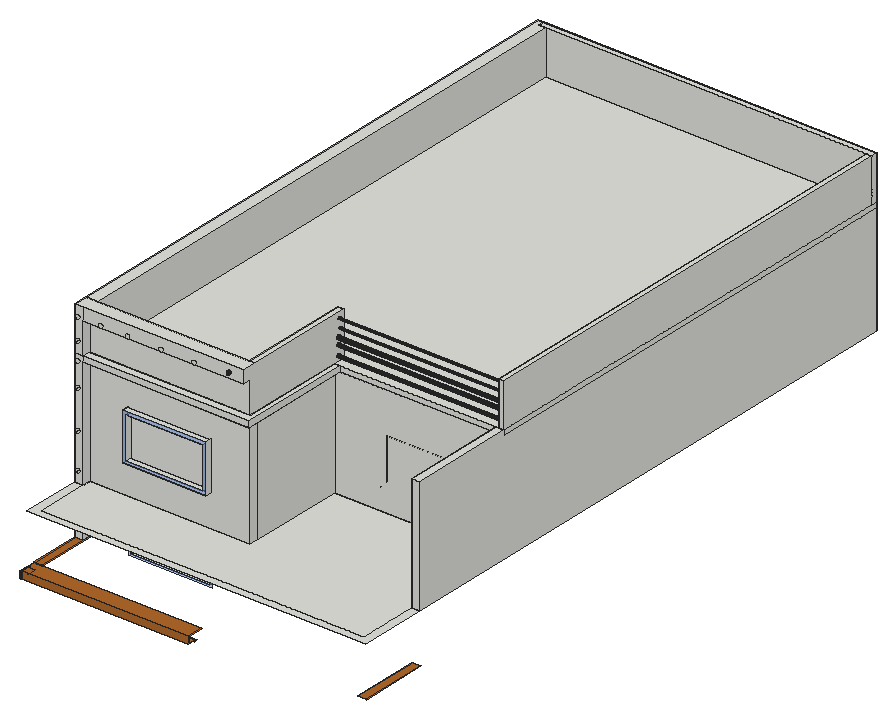
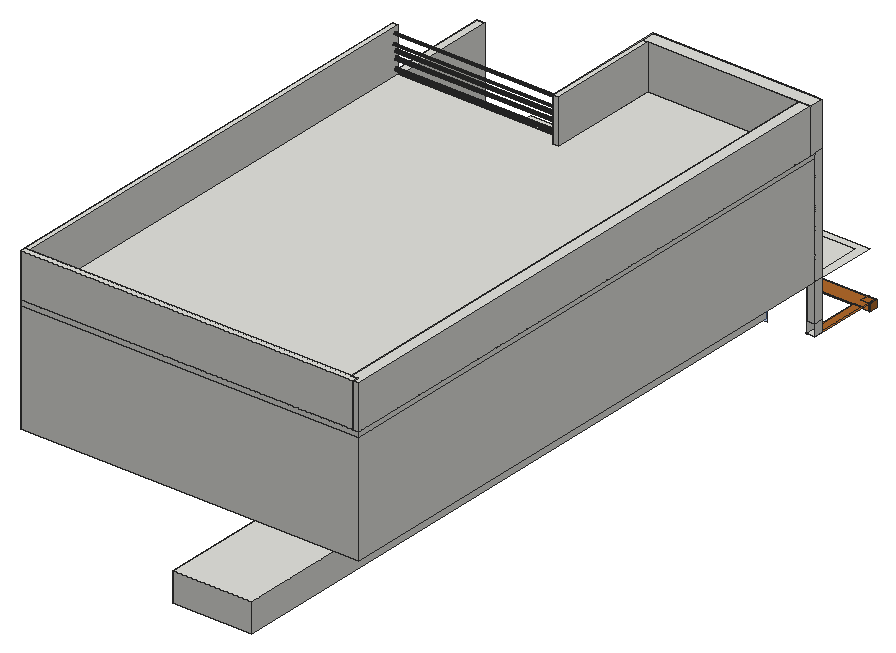
# SketchUp Ruby script. Lengths in inches.
U = 1.inch
M = Sketchup.active_model
def pt(a) = Geom::Point3d.new(a.map { |v| v * U })
def face(e, loops, mat)
  f = e.add_face(loops[0].map { |a| pt(a) })
  loops[1..].each { |l| e.add_face(l.map { |a| pt(a) }).erase! }
  f.material = f.back_material = mat if mat
  f
end
# faces: each face lists its corners as indices into pts; further lists are holes
def faces(e, pts, list, mat = nil) = list.each { |f| face(e, (f[0].is_a?(Array) ? f : [f]).map { |l| l.map { |i| pts[i] } }, mat) }
# xy, xz, yz: faces in a plane at the given z, y or x. An outline is a flat list of corners, or four numbers for a rectangle; further outlines are holes
def ring(l) = l.size == 4 ? [[l[0], l[1]], [l[2], l[1]], [l[2], l[3]], [l[0], l[3]]] : l.each_slice(2).to_a
def flat(e, list, mat, &to3) = list.each { |f| face(e, (f[0].is_a?(Array) ? f : [f]).map { |l| ring(l).map { |u, v| to3.(u, v) } }, mat) }
def xy(e, z, list, mat = nil) = flat(e, list, mat) { |x, y| [x, y, z] }
def xz(e, y, list, mat = nil) = flat(e, list, mat) { |x, z| [x, y, z] }
def yz(e, x, list, mat = nil) = flat(e, list, mat) { |y, z| [x, y, z] }
def lines(e, pts, list) = list.each { |a, b| e.add_line(pt(pts[a]), pt(pts[b])) }
# prism: a flat outline (further loops are holes) pulled along v
def prism(e, loops, v, mat = nil)
  f = face(e, loops, mat); d = Geom::Vector3d.new(v.map { |x| x * U })
  f.pushpull(f.normal.samedirection?(d) ? d.length : -d.length)
end
def box(e, o, s, mat = nil) = prism(e, [[o, [o[0] + s[0], o[1], o[2]], [o[0] + s[0], o[1] + s[1], o[2]], [o[0], o[1] + s[1], o[2]]]], [0, 0, s[2]], mat)
def at(x, y, z, deg = 0) = Geom::Transformation.translation(pt([x, y, z])) * Geom::Transformation.rotation(ORIGIN, Z_AXIS, deg.degrees)
def axes(o, x, y, z) = Geom::Transformation.new([*x, 0, *y, 0, *z, 0, *pt(o).to_a, 1])
def part(name) = M.definitions.add(name)
# library, detail: a bought-in or finely detailed component or shape, given as its bounding box
def library(name, o, s) = part(name).tap { |d| box(d.entities, o, s) }
def detail(e, o, s) = box(e.add_group.entities, o, s)
def put(e, d, t, mat = nil) = e.add_instance(d, t).tap { |i| i.material = mat if mat }
def group(e, t, mat = nil) = e.add_group.tap { |g| g.transformation = t; g.material = mat if mat }.entities
root = M.entities
M.materials.add("[Translucent Glass Blue]").color = [100, 149, 237]
M.materials["[Translucent Glass Blue]"].alpha = 0.5
M.materials.add("[Wood Bamboo]").color = [177, 105, 43]
c1 = part("Component\#1")
xy(c1.entities,0,[[0,0,369,0,369,74,360,74,360,9,9,9,9,74,0,74],[9,9,360,9,360,189,184,189,184,74,9,74],[0,74,184,74,184,83,9,83,9,687,360,687,360,198,175.5625,198,175.5625,189,360,189,360,74,369,74,369,696,0,696],[9,83,175,83,175,198,360,198,360,687,9,687],[175,189,175.5625,198]])
xy(c1.entities,120,[[0,74,184,83],[0,83,9,189],[9,83,9,687,360,687,360,198,175.5625,198,175.5625,189,175,189,175,83],[0,189,9,696],[175.5625,189,369,198],
  [360,198,369,696],[9,687,360,696]])
xy(c1.entities,126,[[0,74,184,74,184,189,369,189,369,696,0,696],[360,74,369,189]])
xz(c1.entities,74,[[0,0,9,120],[9,0,184,120],[360,0,369,126],[0,120,184,126]])
xz(c1.entities,83,[[9,0,175,120],[175,0,184,120]])
xz(c1.entities,189,[[175,0,175.5625,120],[175.5625,0,184,120],[184,0,360,120],[184,120,360,126],[360,120,369,126]])
xz(c1.entities,198,[[175.5625,0,360,120]])
xz(c1.entities,687,[[9,0,360,120]])
xz(c1.entities,696,[[0,0,369,120],[0,120,369,126]])
yz(c1.entities,0,[[74,0,696,120],[74,120,696,126]])
yz(c1.entities,9,[[83,0,687,120]])
yz(c1.entities,175,[[83,0,189,120]])
yz(c1.entities,175.5625,[[189,0,198,120]])
yz(c1.entities,184,[[74,0,83,120],[83,0,189,120],[74,120,189,126]])
yz(c1.entities,360,[[74,0,189,126],[198,0,687,120]])
yz(c1.entities,369,[[74,0,696,0,696,120,189,120,189,126,74,126],[189,120,696,126]])
xy(root,62.76,[[157.01,36.81,183.01,40.24]],"[Wood Bamboo]")
xy(root,64.47,[[0.51,27.81,1.51,36.81],[1.51,27.81,1.51,36.81,83.28,36.81,83.28,45.81,141.28,45.81,141.28,36.81,183.01,36.81,183.01,27.81],[183.01,27.81,184.01,36.81],[82.28,36.81,83.28,45.81],[141.28,36.81,142.28,45.81]],"[Wood Bamboo]")
xy(root,70.55,[[54.61,110.81,140.53,811.24]])
xy(root,72,[[9.45,27.57,9.45,27.59,1.39,27.81,0.51,27.81,0.51,36.81,0.27,27.8125],[10.45,27.57,10.45,27.81,9.45,27.81,9.45,27.59],[9.45,27.59,9.45,27.81,1.39,27.81],[0.51,27.81,1.39,27.81,1.27,27.8125,1.51,36.78,0.51,36.81],[1.39,27.81,1.51,27.81,1.51,36.78,1.27,27.8125],
  [1.51,27.81,9.45,27.81,9.6875,36.5625,1.51,36.78],[10.45,27.81,183.01,27.81,183.01,45.81,1.51,45.81,1.51,36.81,10.6875,36.5625],[9.45,27.81,10.45,27.81,10.6875,36.5625,1.51,36.81,1.51,36.78,9.6875,36.5625],[183.01,27.81,184.01,45.81],[1.51,36.78,1.51,45.81,0.51,45.81,0.51,36.81],
  [360.51,36.81,361.51,110.81],[361.51,36.81,369.51,110.81],[369.51,36.81,370.51,110.81]],"[Wood Bamboo]")
xy(root,72.3125,[[0.51,45.81,1.51,110.81],[1.51,45.81,9.51,110.81],[9.51,45.81,10.51,110.81]],"[Wood Bamboo]")
xy(root,72.54,[[0.51,101.81,9.51,110.81]])
xy(root,84.53,[[0.51,101.81,9.51,110.81]])
xy(root,102.16,[[54.61,110.81,140.53,811.24]])
xy(root,125.75,[[0.51,101.81,9.51,110.81]])
xy(root,126,[[0.51,101.81,9.51,110.81]])
xy(root,156.23,[[241.98,225.81,319.92,292.56]])
xy(root,160.68,[[50.59,104.68,141.46,172.06]])
xy(root,164.35,[[54.26,104.68,137.79,696.81]])
xy(root,201.73,[[241.98,225.81,319.92,292.56]])
xy(root,209.32,[[54.26,104.68,137.79,696.81]])
xy(root,212.99,[[50.59,104.68,141.46,172.06]])
xy(root,246,[[9.51,101.81,190.64,110.81],[184.51,110.81,190.64,225.81]])
xy(root,252,[[0.51,101.81,0.51,116.96,184.51,116.96,184.51,110.81,9.51,110.81,9.51,101.81],[9.51,101.81,190.64,101.81,190.64,225.81,184.51,225.81,184.51,110.81,9.51,110.81],[0.51,116.96,0.51,732.81,6.51,732.81,6.51,726.81,13.58,726.81,13.58,116.96],[178.51,116.96,184.51,237.875],[363.51,225.81,369.51,726.81],
  [6.51,726.81,369.51,732.81]])
xy(root,286.07,[[9.51,101.81,184.51,110.81]])
xy(root,300,[[0.51,101.81,184.51,116.96],[0.51,116.96,13.58,116.96,13.58,726.81,6.51,726.81,6.51,732.81,0.51,732.81],[178.51,116.96,184.51,237.875],[363.51,225.81,369.51,726.81],[6.51,726.81,369.51,732.81]])
xz(root,27.81,[[0.51,64.47,1.51,72],[1.51,64.47,183.01,72],[183.01,64.47,184.01,72]],"[Wood Bamboo]")
xz(root,45.81,[[0.51,72,1.51,72.3125],[1.51,72,9.51,72.3125],[9.51,72,10.51,72.3125]],"[Wood Bamboo]")
xz(root,96.37,[[[7.9375,84.47,8.45,84.53,8.9375,84.73,9.35,85.05,9.67,85.47,9.87,85.95,9.9375,86.47,9.87,86.98,9.67,87.47,9.35,87.88,8.9375,88.2,8.45,88.4,7.9375,88.47,7.42,88.4,6.9375,88.2,6.52,87.88,6.2,87.47,6.01,86.98,5.9375,86.47,6.01,85.95,6.2,85.47,6.52,85.05,6.9375,84.73,7.42,84.53],[7.9375,85.47,7.68,85.5,7.4375,85.6,7.23,85.76,7.07,85.97,6.97,86.21,6.9375,86.47,6.97,86.72,7.07,86.97,7.23,87.17,7.4375,87.33,7.68,87.43,7.9375,87.47,8.2,87.43,8.4375,87.33,8.64,87.17,8.8,86.97,8.9,86.72,8.9375,86.47,8.9,86.21,8.8,85.97,8.64,85.76,8.4375,85.6,8.2,85.5]],[[7.9375,113.05,8.45,113.12,8.9375,113.32,9.35,113.64,9.67,114.05,9.87,114.54,9.9375,115.05,9.87,115.57,9.67,116.05,9.35,116.47,8.9375,116.79,8.45,116.99,7.9375,117.05,7.42,116.99,6.9375,116.79,6.52,116.47,6.2,116.05,6.01,115.57,5.9375,115.05,6.01,114.54,6.2,114.05,6.52,113.64,6.9375,113.32,7.42,113.12],[7.9375,114.05,7.68,114.09,7.4375,114.1875,7.23,114.35,7.07,114.55,6.97,114.8,6.9375,115.05,6.97,115.3125,7.07,115.55,7.23,115.76,7.4375,115.92,7.68,116.02,7.9375,116.05,8.2,116.02,8.4375,115.92,8.64,115.76,8.8,115.55,8.9,115.3125,8.9375,115.05,8.9,114.8,8.8,114.55,8.64,114.35,8.4375,114.1875,8.2,114.09]],[[7.9375,140.18,8.45,140.25,8.9375,140.45,9.35,140.77,9.67,141.18,9.87,141.66,9.9375,142.18,9.87,142.7,9.67,143.18,9.35,143.59,8.9375,143.91,8.45,144.11,7.9375,144.18,7.42,144.11,6.9375,143.91,6.52,143.59,6.2,143.18,6.01,142.7,5.9375,142.18,6.01,141.66,6.2,141.18,6.52,140.77,6.9375,140.45,7.42,140.25],[7.9375,141.18,7.68,141.21,7.4375,141.3125,7.23,141.47,7.07,141.68,6.97,141.92,6.9375,142.18,6.97,142.4375,7.07,142.68,7.23,142.89,7.4375,143.05,7.68,143.15,7.9375,143.18,8.2,143.15,8.4375,143.05,8.64,142.89,8.8,142.68,8.9,142.4375,8.9375,142.18,8.9,141.92,8.8,141.68,8.64,141.47,8.4375,141.3125,8.2,141.21]],[[7.9375,179.1,8.45,179.17,8.9375,179.37,9.35,179.69,9.67,180.1,9.87,180.59,9.9375,181.1,9.87,181.62,9.67,182.1,9.35,182.52,8.9375,182.84,8.45,183.04,7.9375,183.1,7.42,183.04,6.9375,182.84,6.52,182.52,6.2,182.1,6.01,181.62,5.9375,181.1,6.01,180.59,6.2,180.1,6.52,179.69,6.9375,179.37,7.42,179.17],[7.9375,180.1,7.68,180.14,7.4375,180.24,7.23,180.4,7.07,180.6,6.97,180.85,6.9375,181.1,6.97,181.36,7.07,181.6,7.23,181.8125,7.4375,181.97,7.68,182.07,7.9375,182.1,8.2,182.07,8.4375,181.97,8.64,181.8125,8.8,181.6,8.9,181.36,8.9375,181.1,8.9,180.85,8.8,180.6,8.64,180.4,8.4375,180.24,8.2,180.14]],[[7.9375,221.04,8.45,221.11,8.9375,221.31,9.35,221.63,9.67,222.04,9.87,222.52,9.9375,223.04,9.87,223.56,9.67,224.04,9.35,224.46,8.9375,224.77,8.45,224.97,7.9375,225.04,7.42,224.97,6.9375,224.77,6.52,224.46,6.2,224.04,6.01,223.56,5.9375,223.04,6.01,222.52,6.2,222.04,6.52,221.63,6.9375,221.31,7.42,221.11],[7.9375,222.04,7.68,222.08,7.4375,222.18,7.23,222.34,7.07,222.54,6.97,222.78,6.9375,223.04,6.97,223.3,7.07,223.54,7.23,223.75,7.4375,223.91,7.68,224.01,7.9375,224.04,8.2,224.01,8.4375,223.91,8.64,223.75,8.8,223.54,8.9,223.3,8.9375,223.04,8.9,222.78,8.8,222.54,8.64,222.34,8.4375,222.18,8.2,222.08]],
  [[7.9375,247.17,8.45,247.24,8.9375,247.44,9.35,247.75,9.67,248.17,9.87,248.65,9.9375,249.17,9.87,249.68,9.67,250.17,9.35,250.58,8.9375,250.9,8.45,251.1,7.9375,251.17,7.42,251.1,6.9375,250.9,6.52,250.58,6.2,250.17,6.01,249.68,5.9375,249.17,6.01,248.65,6.2,248.17,6.52,247.75,6.9375,247.44,7.42,247.24],[7.9375,248.17,7.68,248.2,7.4375,248.3,7.23,248.46,7.07,248.67,6.97,248.91,6.9375,249.17,6.97,249.43,7.07,249.67,7.23,249.875,7.4375,250.03,7.68,250.13,7.9375,250.17,8.2,250.13,8.4375,250.03,8.64,249.875,8.8,249.67,8.9,249.43,8.9375,249.17,8.9,248.91,8.8,248.67,8.64,248.46,8.4375,248.3,8.2,248.2]],[[7.92,267.07,8.4375,267.14,8.92,267.34,9.33,267.65,9.65,268.07,9.85,268.55,9.92,269.07,9.85,269.59,9.65,270.07,9.33,270.48,8.92,270.8,8.4375,271,7.92,271.07,7.4,271,6.92,270.8,6.51,270.48,6.1875,270.07,5.99,269.59,5.92,269.07,5.99,268.55,6.1875,268.07,6.51,267.65,6.92,267.34,7.4,267.14],[7.92,268.07,7.66,268.1,7.42,268.2,7.21,268.36,7.05,268.57,6.95,268.81,6.92,269.07,6.95,269.33,7.05,269.57,7.21,269.78,7.42,269.93,7.66,270.03,7.92,270.07,8.18,270.03,8.42,269.93,8.63,269.78,8.79,269.57,8.89,269.33,8.92,269.07,8.89,268.81,8.79,268.57,8.63,268.36,8.42,268.2,8.18,268.1]],[[7.92,290.19,8.4375,290.26,8.92,290.46,9.33,290.78,9.65,291.19,9.85,291.68,9.92,292.19,9.85,292.71,9.65,293.19,9.33,293.61,8.92,293.93,8.4375,294.125,7.92,294.19,7.4,294.125,6.92,293.93,6.51,293.61,6.1875,293.19,5.99,292.71,5.92,292.19,5.99,291.68,6.1875,291.19,6.51,290.78,6.92,290.46,7.4,290.26],[7.92,291.19,7.66,291.23,7.42,291.33,7.21,291.49,7.05,291.69,6.95,291.93,6.92,292.19,6.95,292.45,7.05,292.69,7.21,292.9,7.42,293.06,7.66,293.16,7.92,293.19,8.18,293.16,8.42,293.06,8.63,292.9,8.79,292.69,8.89,292.45,8.92,292.19,8.89,291.93,8.79,291.69,8.63,291.49,8.42,291.33,8.18,291.23]],[[32.92,290.19,33.4375,290.26,33.92,290.46,34.33,290.78,34.65,291.19,34.85,291.68,34.92,292.19,34.85,292.71,34.65,293.19,34.33,293.61,33.92,293.93,33.4375,294.125,32.92,294.19,32.4,294.125,31.92,293.93,31.51,293.61,31.1875,293.19,30.99,292.71,30.92,292.19,30.99,291.68,31.1875,291.19,31.51,290.78,31.92,290.46,32.4,290.26],[32.92,291.19,32.66,291.23,32.42,291.33,32.21,291.49,32.05,291.69,31.95,291.93,31.92,292.19,31.95,292.45,32.05,292.69,32.21,292.9,32.42,293.06,32.66,293.16,32.92,293.19,33.18,293.16,33.42,293.06,33.63,292.9,33.79,292.69,33.89,292.45,33.92,292.19,33.89,291.93,33.79,291.69,33.63,291.49,33.42,291.33,33.18,291.23]],[[62.18,290.19,62.69,290.26,63.18,290.46,63.59,290.78,63.91,291.19,64.11,291.68,64.18,292.19,64.11,292.71,63.91,293.19,63.59,293.61,63.18,293.93,62.69,294.125,62.18,294.19,61.66,294.125,61.18,293.93,60.76,293.61,60.44,293.19,60.24,292.71,60.18,292.19,60.24,291.68,60.44,291.19,60.76,290.78,61.18,290.46,61.66,290.26],[62.18,291.19,61.92,291.23,61.68,291.33,61.47,291.49,61.31,291.69,61.21,291.93,61.18,292.19,61.21,292.45,61.31,292.69,61.47,292.9,61.68,293.06,61.92,293.16,62.18,293.19,62.43,293.16,62.68,293.06,62.88,292.9,63.04,292.69,63.14,292.45,63.18,292.19,63.14,291.93,63.04,291.69,62.88,291.49,62.68,291.33,62.43,291.23]],
  [[98.61,290.19,99.13,290.26,99.61,290.46,100.03,290.78,100.35,291.19,100.55,291.68,100.61,292.19,100.55,292.71,100.35,293.19,100.03,293.61,99.61,293.93,99.13,294.125,98.61,294.19,98.1,294.125,97.61,293.93,97.2,293.61,96.88,293.19,96.68,292.71,96.61,292.19,96.68,291.68,96.88,291.19,97.2,290.78,97.61,290.46,98.1,290.26],[98.61,291.19,98.35,291.23,98.11,291.33,97.91,291.49,97.75,291.69,97.65,291.93,97.61,292.19,97.65,292.45,97.75,292.69,97.91,292.9,98.11,293.06,98.35,293.16,98.61,293.19,98.87,293.16,99.11,293.06,99.32,292.9,99.48,292.69,99.58,292.45,99.61,292.19,99.58,291.93,99.48,291.69,99.32,291.49,99.11,291.33,98.87,291.23]],[[134.8,290.19,135.31,290.26,135.8,290.46,136.21,290.78,136.53,291.19,136.73,291.68,136.8,292.19,136.73,292.71,136.53,293.19,136.21,293.61,135.8,293.93,135.31,294.125,134.8,294.19,134.28,294.125,133.8,293.93,133.38,293.61,133.07,293.19,132.87,292.71,132.8,292.19,132.87,291.68,133.07,291.19,133.38,290.78,133.8,290.46,134.28,290.26],[134.8,291.19,134.54,291.23,134.3,291.33,134.09,291.49,133.93,291.69,133.83,291.93,133.8,292.19,133.83,292.45,133.93,292.69,134.09,292.9,134.3,293.06,134.54,293.16,134.8,293.19,135.06,293.16,135.3,293.06,135.5,292.9,135.66,292.69,135.76,292.45,135.8,292.19,135.76,291.93,135.66,291.69,135.5,291.49,135.3,291.33,135.06,291.23]]])
xz(root,100.24,[[[168.98,290.19,169.5,290.26,169.98,290.46,170.4,290.78,170.72,291.19,170.92,291.68,170.98,292.19,170.92,292.71,170.72,293.19,170.4,293.61,169.98,293.93,169.5,294.125,168.98,294.19,168.47,294.125,167.98,293.93,167.57,293.61,167.25,293.19,167.05,292.71,166.98,292.19,167.05,291.68,167.25,291.19,167.57,290.78,167.98,290.46,168.47,290.26],[168.98,291.19,168.73,291.23,168.48,291.33,168.28,291.49,168.12,291.69,168.02,291.93,167.98,292.19,168.02,292.45,168.12,292.69,168.28,292.9,168.48,293.06,168.73,293.16,168.98,293.19,169.24,293.16,169.48,293.06,169.69,292.9,169.85,292.69,169.95,292.45,169.98,292.19,169.95,291.93,169.85,291.69,169.69,291.49,169.48,291.33,169.24,291.23]]])
xz(root,101.81,[[0.51,72.54,9.51,84.53],[0.51,84.53,9.51,125.75],[0.51,126,9.51,252],[9.51,246,190.64,252],[0.51,252,9.51,300],
  [[9.51,286.07,184.51,300],[168.98,290.19,168.47,290.26,167.98,290.46,167.57,290.78,167.25,291.19,167.05,291.68,166.98,292.19,167.05,292.71,167.25,293.19,167.57,293.61,167.98,293.93,168.47,294.125,168.98,294.19,169.5,294.125,169.98,293.93,170.4,293.61,170.72,293.19,170.92,292.71,170.98,292.19,170.92,291.68,170.72,291.19,170.4,290.78,169.98,290.46,169.5,290.26]],[168.98,291.19,169.24,291.23,169.48,291.33,169.69,291.49,169.85,291.69,169.95,291.93,169.98,292.19,169.95,292.45,169.85,292.69,169.69,292.9,169.48,293.06,169.24,293.16,168.98,293.19,168.73,293.16,168.48,293.06,168.28,292.9,168.12,292.69,168.02,292.45,167.98,292.19,168.02,291.93,168.12,291.69,168.28,291.49,168.48,291.33,168.73,291.23]])
xz(root,104.68,[[[50.59,160.68,141.46,212.99],[54.26,164.35,137.79,209.32]]],"[Translucent Glass Blue]")
xz(root,110.81,[[0.51,84.53,9.51,125.75],[9.51,252,184.51,286.07]])
xz(root,110.81,[[[51.66,67.6,143.47,105.1],[54.61,70.55,140.53,102.16]]],"[Translucent Glass Blue]")
xz(root,116.96,[[0.51,252,13.58,300],[13.58,252,178.51,300]])
xz(root,172.06,[[50.59,160.68,141.46,212.99]])
xz(root,225.81,[[[235.11,149.36,326.8,208.61],[241.98,156.23,319.92,201.73]],[184.51,246,190.64,252],[363.51,252,369.51,300]])
xz(root,237.875,[[178.51,252,184.51,300]])
xz(root,292.56,[[241.98,156.23,319.92,201.73]])
xz(root,696.81,[[[54.26,164.35,137.79,209.32],[74.57,184.66,117.48,189.01]],[74.57,184.66,117.48,189.01]])
xz(root,726.81,[[6.51,252,13.58,300],[13.58,252,363.51,300],[363.51,252,369.51,300]])
xz(root,732.81,[[0.51,252,6.51,300],[6.51,252,369.51,300]])
xz(root,811.24,[[54.61,70.55,140.53,102.16]])
yz(root,0.51,[[101.81,72.54,110.81,84.53],[101.81,84.53,110.81,125.75],[101.81,126,110.81,252],[101.81,252,116.96,300],[116.96,252,732.81,300]])
yz(root,0.51,[[27.81,64.47,36.81,72]],"[Wood Bamboo]")
yz(root,1.51,[[27.81,64.47,36.81,72]],"[Wood Bamboo]")
yz(root,6.51,[[726.81,252,732.81,300]])
yz(root,9.51,[[101.81,72.54,110.81,84.53],[101.81,84.53,110.81,125.75],[101.81,126,110.81,246],[101.81,252,110.81,286.07]])
yz(root,13.58,[[116.96,252,726.81,300]])
yz(root,50.59,[[104.68,160.68,172.06,212.99]])
yz(root,54.26,[[104.68,164.35,696.81,209.32]])
yz(root,54.61,[[110.81,70.55,811.24,102.16]])
yz(root,137.79,[[104.68,164.35,696.81,209.32]])
yz(root,140.53,[[110.81,70.55,811.24,102.16]])
yz(root,141.46,[[104.68,160.68,172.06,212.99]])
yz(root,178.51,[[116.96,252,237.875,300]])
yz(root,184.26,[[231.02,293.29,230.76,293.33,230.52,293.43,230.3125,293.58,230.15,293.79,230.05,294.03,230.02,294.29,230.05,294.55,230.15,294.79,230.3125,295,230.52,295.16,230.76,295.26,231.02,295.29,231.28,295.26,231.52,295.16,231.73,295,231.89,294.79,231.99,294.55,232.02,294.29,231.99,294.03,231.89,293.79,231.73,293.58,231.52,293.43,231.28,293.33]])
yz(root,184.51,[[[110.81,252,237.875,252,237.875,300,101.81,300,101.81,286.07,110.81,286.07],[232.27,283.2,232.01,283.23,231.76,283.32,231.55,283.47,231.39,283.67,231.28,283.91,231.24,284.17,231.26,284.43,231.35,284.67,231.5,284.88,231.71,285.05,231.94,285.16,232.2,285.2,232.46,285.17,232.71,285.08,232.92,284.93,233.08,284.73,233.19,284.49,233.23,284.23,233.21,283.97,233.12,283.73,232.97,283.52,232.76,283.35,232.53,283.24]]])
yz(root,190.64,[[101.81,246,225.81,252]])
yz(root,241.98,[[225.81,156.23,292.56,201.73]])
yz(root,319.92,[[225.81,156.23,292.56,201.73]])
yz(root,363.51,[[[225.81,252,726.81,300],[232.27,283.2,232.53,283.24,232.76,283.35,232.97,283.52,233.12,283.73,233.21,283.97,233.23,284.23,233.19,284.49,233.08,284.73,232.92,284.93,232.71,285.08,232.46,285.17,232.2,285.2,231.94,285.16,231.71,285.05,231.5,284.88,231.35,284.67,231.26,284.43,231.24,284.17,231.28,283.91,231.39,283.67,231.55,283.47,231.76,283.32,232.01,283.23],[231.02,293.29,231.28,293.33,231.52,293.43,231.73,293.58,231.89,293.79,231.99,294.03,232.02,294.29,231.99,294.55,231.89,294.79,231.73,295,231.52,295.16,231.28,295.26,231.02,295.29,230.76,295.26,230.52,295.16,230.3125,295,230.15,294.79,230.05,294.55,230.02,294.29,230.05,294.03,230.15,293.79,230.3125,293.58,230.52,293.43,230.76,293.33]]])
yz(root,369.51,[[225.81,252,726.81,300],[726.81,252,732.81,300]])
p = [[0.51,36.81,72],[0.51,36.81,64.47],[0.27,27.8125,64.47],[0.27,27.8125,72],[1.51,36.81,72],[1.51,36.81,64.47],
  [1.27,27.8125,64.47],[1.27,27.8125,72],[1.51,36.78,72],[363.51,228.86,257.03],[363.51,228.48,257.19],[184.51,228.48,257.19],
  [184.51,228.86,257.03],[363.51,229.26,256.98],[184.51,229.26,256.98],[363.51,229.67,257.03],[184.51,229.67,257.03],[363.51,230.05,257.19],
  [184.51,230.05,257.19],[363.51,228.16,257.4375],[184.51,228.16,257.4375],[363.51,230.37,257.4375],[184.51,230.37,257.4375],[363.51,227.91,257.76],
  [184.51,227.91,257.76],[363.51,230.62,257.76],[184.51,230.62,257.76],[363.51,227.76,258.14],[184.51,227.76,258.14],[363.51,230.77,258.14],
  [184.51,230.77,258.14],[363.51,227.7,258.54],[184.51,227.7,258.54],[363.51,230.83,258.54],[184.51,230.83,258.54],[363.51,227.76,258.95],
  [184.51,227.76,258.95],[363.51,230.77,258.95],[184.51,230.77,258.95],[363.51,227.91,259.32],[184.51,227.91,259.32],[363.51,230.62,259.32],
  [184.51,230.62,259.32],[363.51,228.16,259.65],[184.51,228.16,259.65],[363.51,230.37,259.65],[184.51,230.37,259.65],[363.51,228.48,259.9],
  [184.51,228.48,259.9],[363.51,230.05,259.9],[184.51,230.05,259.9],[363.51,228.86,260.05],[184.51,228.86,260.05],[363.51,229.67,260.05],
  [184.51,229.67,260.05],[363.51,229.26,260.11],[184.51,229.26,260.11],[363.51,229.26,267.42],[363.51,228.86,267.47],[184.51,228.86,267.47],
  [184.51,229.26,267.42],[363.51,229.67,267.47],[184.51,229.67,267.47],[363.51,228.48,267.63],[184.51,228.48,267.63],[363.51,230.05,267.63],
  [184.51,230.05,267.63],[363.51,228.16,267.875],[184.51,228.16,267.875],[363.51,230.37,267.875],[184.51,230.37,267.875],[363.51,227.91,268.2],
  [184.51,227.91,268.2],[363.51,230.62,268.2],[184.51,230.62,268.2],[363.51,227.76,268.58],[184.51,227.76,268.58],[363.51,230.77,268.58],
  [184.51,230.77,268.58],[363.51,227.7,268.98],[184.51,227.7,268.98],[363.51,230.83,268.98],[184.51,230.83,268.98],[363.51,227.76,269.38],
  [184.51,227.76,269.38],[363.51,230.77,269.38],[184.51,230.77,269.38],[363.51,227.91,269.76],[184.51,227.91,269.76],[363.51,230.62,269.76],
  [184.51,230.62,269.76],[363.51,228.16,270.09],[184.51,228.16,270.09],[363.51,230.37,270.09],[184.51,230.37,270.09],[363.51,228.48,270.33],
  [184.51,228.48,270.33],[363.51,230.05,270.33],[184.51,230.05,270.33],[363.51,228.86,270.49],[184.51,228.86,270.49],[363.51,229.67,270.49],
  [184.51,229.67,270.49],[363.51,229.26,270.54],[184.51,229.26,270.54],[363.51,229.26,274.73],[363.51,228.86,274.78],[184.51,228.86,274.78],
  [184.51,229.26,274.73],[363.51,229.67,274.78],[184.51,229.67,274.78],[363.51,228.48,274.94],[184.51,228.48,274.94],[363.51,230.05,274.94],
  [184.51,230.05,274.94],[363.51,228.16,275.1875],[184.51,228.16,275.1875],[363.51,230.37,275.1875],[184.51,230.37,275.1875],[363.51,227.91,275.51],
  [184.51,227.91,275.51],[363.51,230.62,275.51],[184.51,230.62,275.51],[363.51,227.76,275.89],[184.51,227.76,275.89],[363.51,230.77,275.89],
  [184.51,230.77,275.89],[363.51,227.7,276.29],[184.51,227.7,276.29],[363.51,230.83,276.29],[184.51,230.83,276.29],[363.51,227.76,276.7],
  [184.51,227.76,276.7],[363.51,230.77,276.7],[184.51,230.77,276.7],[363.51,227.91,277.07],[184.51,227.91,277.07],[363.51,230.62,277.07],
  [184.51,230.62,277.07],[363.51,228.16,277.4],[184.51,228.16,277.4],[363.51,230.37,277.4],[184.51,230.37,277.4],[363.51,228.48,277.65],
  [184.51,228.48,277.65],[363.51,230.05,277.65],[184.51,230.05,277.65],[363.51,228.86,277.8],[184.51,228.86,277.8],[363.51,229.67,277.8],
  [184.51,229.67,277.8],[363.51,229.26,277.86],[184.51,229.26,277.86],[184.51,231.76,283.32],[184.51,232.01,283.23],[363.51,232.01,283.23],
  [363.51,231.76,283.32],[184.51,232.27,283.2],[363.51,232.27,283.2],[184.51,232.53,283.24],[363.51,232.53,283.24],[184.51,232.76,283.35],
  [363.51,232.76,283.35],[184.51,231.55,283.47],[363.51,231.55,283.47],[184.51,232.97,283.52],[363.51,232.97,283.52],[184.51,231.39,283.67],
  [363.51,231.39,283.67],[184.51,233.12,283.73],[363.51,233.12,283.73],[184.51,231.28,283.91],[363.51,231.28,283.91],[184.51,233.21,283.97],
  [363.51,233.21,283.97],[184.51,231.24,284.17],[363.51,231.24,284.17],[184.51,233.23,284.23],[363.51,233.23,284.23],[184.51,231.26,284.43],
  [363.51,231.26,284.43],[184.51,233.19,284.49],[363.51,233.19,284.49],[184.51,231.35,284.67],[363.51,231.35,284.67],[184.51,233.08,284.73],
  [363.51,233.08,284.73],[184.51,231.5,284.88],[363.51,231.5,284.88],[184.51,232.92,284.93],[363.51,232.92,284.93],[184.51,231.71,285.05],
  [363.51,231.71,285.05],[184.51,232.71,285.08],[363.51,232.71,285.08],[184.51,231.94,285.16],[363.51,231.94,285.16],[184.51,232.46,285.17],
  [363.51,232.46,285.17],[184.51,232.2,285.2],[363.51,232.2,285.2],[168.47,101.81,290.26],[168.98,101.81,290.19],[168.98,100.24,290.19],
  [168.47,100.24,290.26],[169.5,101.81,290.26],[169.5,100.24,290.26],[167.98,101.81,290.46],[167.98,100.24,290.46],[169.98,101.81,290.46],
  [169.98,100.24,290.46],[167.57,101.81,290.78],[167.57,100.24,290.78],[170.4,101.81,290.78],[170.4,100.24,290.78],[167.25,101.81,291.19],
  [167.25,100.24,291.19],[170.72,101.81,291.19],[170.72,100.24,291.19],[167.05,101.81,291.68],[167.05,100.24,291.68],[168.73,101.81,291.23],
  [168.48,101.81,291.33],[168.48,100.24,291.33],[168.73,100.24,291.23],[168.98,101.81,291.19],[168.98,100.24,291.19],[169.24,101.81,291.23],
  [169.24,100.24,291.23],[169.48,101.81,291.33],[169.48,100.24,291.33],[170.92,101.81,291.68],[170.92,100.24,291.68],[168.28,101.81,291.49],
  [168.28,100.24,291.49],[169.69,101.81,291.49],[169.69,100.24,291.49],[168.12,101.81,291.69],[168.12,100.24,291.69],[169.85,101.81,291.69],
  [169.85,100.24,291.69],[166.98,101.81,292.19],[166.98,100.24,292.19],[168.02,101.81,291.93],[168.02,100.24,291.93],[169.95,101.81,291.93],
  [169.95,100.24,291.93],[170.98,101.81,292.19],[170.98,100.24,292.19],[167.98,101.81,292.19],[167.98,100.24,292.19],[169.98,101.81,292.19],
  [169.98,100.24,292.19],[167.05,101.81,292.71],[167.05,100.24,292.71],[168.02,101.81,292.45],[168.02,100.24,292.45],[169.95,101.81,292.45],
  [169.95,100.24,292.45],[170.92,101.81,292.71],[170.92,100.24,292.71],[168.12,101.81,292.69],[168.12,100.24,292.69],[169.85,101.81,292.69],
  [169.85,100.24,292.69],[167.25,101.81,293.19],[167.25,100.24,293.19],[168.28,101.81,292.9],[168.28,100.24,292.9],[169.69,101.81,292.9],
  [169.69,100.24,292.9],[170.72,101.81,293.19],[170.72,100.24,293.19],[168.48,101.81,293.06],[168.48,100.24,293.06],[169.48,101.81,293.06],
  [169.48,100.24,293.06],[168.73,101.81,293.16],[168.73,100.24,293.16],[169.24,101.81,293.16],[169.24,100.24,293.16],[167.57,101.81,293.61],
  [167.57,100.24,293.61],[168.98,101.81,293.19],[168.98,100.24,293.19],[170.4,101.81,293.61],[170.4,100.24,293.61],[363.51,230.76,293.33],
  [363.51,230.52,293.43],[184.26,230.52,293.43],[184.26,230.76,293.33],[363.51,231.02,293.29],[184.26,231.02,293.29],[363.51,231.28,293.33],
  [184.26,231.28,293.33],[363.51,231.52,293.43],[184.26,231.52,293.43],[363.51,230.3125,293.58],[184.26,230.3125,293.58],[363.51,231.73,293.58],
  [184.26,231.73,293.58],[167.98,101.81,293.93],[167.98,100.24,293.93],[169.98,101.81,293.93],[169.98,100.24,293.93],[363.51,230.15,293.79],
  [184.26,230.15,293.79],[363.51,231.89,293.79],[184.26,231.89,293.79],[363.51,230.05,294.03],[184.26,230.05,294.03],[363.51,231.99,294.03],
  [184.26,231.99,294.03],[168.47,101.81,294.125],[168.47,100.24,294.125],[169.5,101.81,294.125],[169.5,100.24,294.125],[363.51,230.02,294.29],
  [184.26,230.02,294.29],[363.51,232.02,294.29],[184.26,232.02,294.29],[168.98,101.81,294.19],[168.98,100.24,294.19],[363.51,230.05,294.55],
  [184.26,230.05,294.55],[363.51,231.99,294.55],[184.26,231.99,294.55],[363.51,230.15,294.79],[184.26,230.15,294.79],[363.51,231.89,294.79],
  [184.26,231.89,294.79],[363.51,230.3125,295],[184.26,230.3125,295],[363.51,231.73,295],[184.26,231.73,295],[363.51,230.52,295.16],
  [184.26,230.52,295.16],[363.51,231.52,295.16],[184.26,231.52,295.16],[363.51,230.76,295.26],[184.26,230.76,295.26],[363.51,231.28,295.26],
  [184.26,231.28,295.26],[363.51,231.02,295.29],[184.26,231.02,295.29]]
faces(root,p,[[0,1,2,3],[4,5,6,7,8]],"[Wood Bamboo]")
faces(root,p,[[9,10,11,12],[13,9,12,14],[15,13,14,16],[17,15,16,18],[10,19,20,11],[21,17,18,22],[19,23,24,20],[25,21,22,26],
  [23,27,28,24],[29,25,26,30],[27,31,32,28],[33,29,30,34],[31,35,36,32],[37,33,34,38],[35,39,40,36],[41,37,38,42],
  [39,43,44,40],[45,41,42,46],[43,47,48,44],[49,45,46,50],[47,51,52,48],[53,49,50,54],[51,55,56,52],[55,53,54,56],
  [57,58,59,60],[61,57,60,62],[58,63,64,59],[65,61,62,66],[63,67,68,64],[69,65,66,70],[67,71,72,68],[73,69,70,74],
  [71,75,76,72],[77,73,74,78],[75,79,80,76],[81,77,78,82],[79,83,84,80],[85,81,82,86],[83,87,88,84],[89,85,86,90],
  [87,91,92,88],[93,89,90,94],[91,95,96,92],[97,93,94,98],[95,99,100,96],[101,97,98,102],[99,103,104,100],[103,101,102,104],
  [105,106,107,108],[109,105,108,110],[106,111,112,107],[113,109,110,114],[111,115,116,112],[117,113,114,118],[115,119,120,116],[121,117,118,122],
  [119,123,124,120],[125,121,122,126],[123,127,128,124],[129,125,126,130],[127,131,132,128],[133,129,130,134],[131,135,136,132],[137,133,134,138],
  [135,139,140,136],[141,137,138,142],[139,143,144,140],[145,141,142,146],[143,147,148,144],[149,145,146,150],[147,151,152,148],[151,149,150,152],
  [153,154,155,156],[154,157,158,155],[157,159,160,158],[159,161,162,160],[163,153,156,164],[161,165,166,162],[167,163,164,168],[165,169,170,166],
  [171,167,168,172],[169,173,174,170],[175,171,172,176],[173,177,178,174],[179,175,176,180],[177,181,182,178],[183,179,180,184],[181,185,186,182],
  [187,183,184,188],[185,189,190,186],[191,187,188,192],[189,193,194,190],[195,191,192,196],[193,197,198,194],[199,195,196,200],[197,199,200,198],
  [201,202,203,204],[202,205,206,203],[207,201,204,208],[205,209,210,206],[211,207,208,212],[209,213,214,210],[215,211,212,216],[213,217,218,214],
  [219,215,216,220],[221,222,223,224],[225,221,224,226],[227,225,226,228],[229,227,228,230],[217,231,232,218],[222,233,234,223],[235,229,230,236],
  [233,237,238,234],[239,235,236,240],[241,219,220,242],[237,243,244,238],[245,239,240,246],[231,247,248,232],[243,249,250,244],[251,245,246,252],
  [253,241,242,254],[249,255,256,250],[257,251,252,258],[247,259,260,248],[255,261,262,256],[263,257,258,264],[265,253,254,266],[261,267,268,262],
  [269,263,264,270],[259,271,272,260],[267,273,274,268],[275,269,270,276],[273,277,278,274],[279,275,276,280],[281,265,266,282],[277,283,284,278],
  [283,279,280,284],[271,285,286,272],[287,288,289,290],[291,287,290,292],[293,291,292,294],[295,293,294,296],[288,297,298,289],[299,295,296,300],
  [301,281,282,302],[285,303,304,286],[297,305,306,298],[307,299,300,308],[305,309,310,306],[311,307,308,312],[313,301,302,314],[303,315,316,304],
  [309,317,318,310],[319,311,312,320],[321,313,314,322],[315,321,322,316],[317,323,324,318],[325,319,320,326],[323,327,328,324],[329,325,326,330],
  [327,331,332,328],[333,329,330,334],[331,335,336,332],[337,333,334,338],[335,339,340,336],[341,337,338,342],[339,343,344,340],[343,341,342,344]])
put(root,c1,at(0.51,36.81,126))
